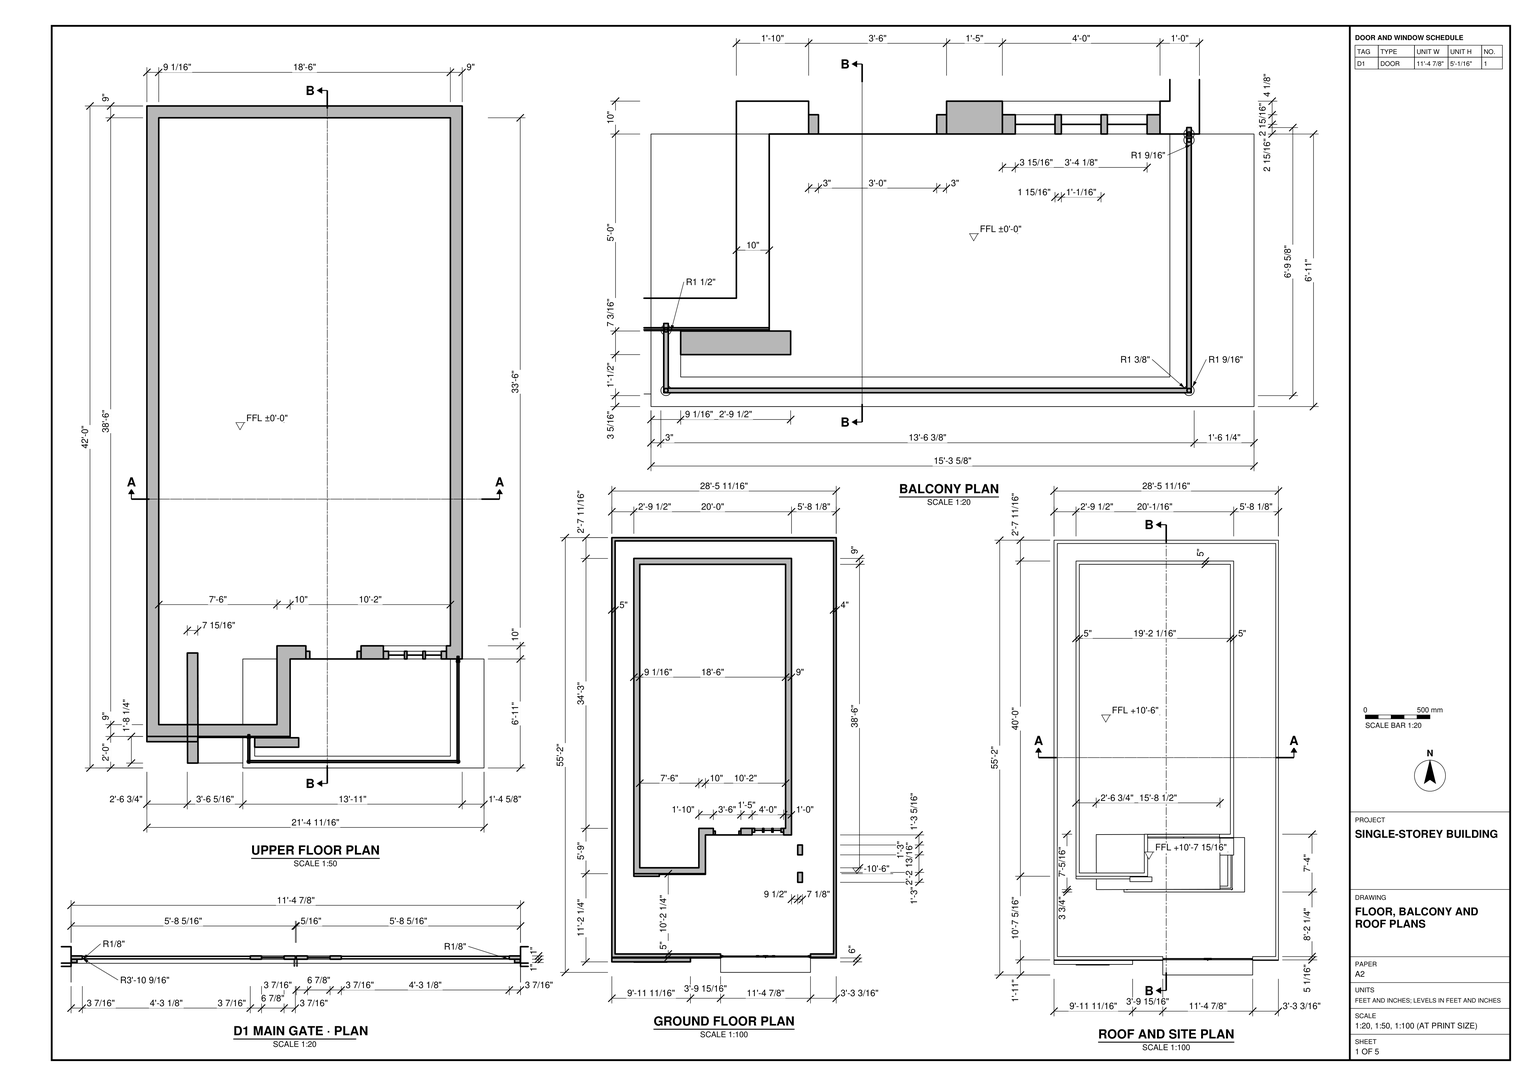
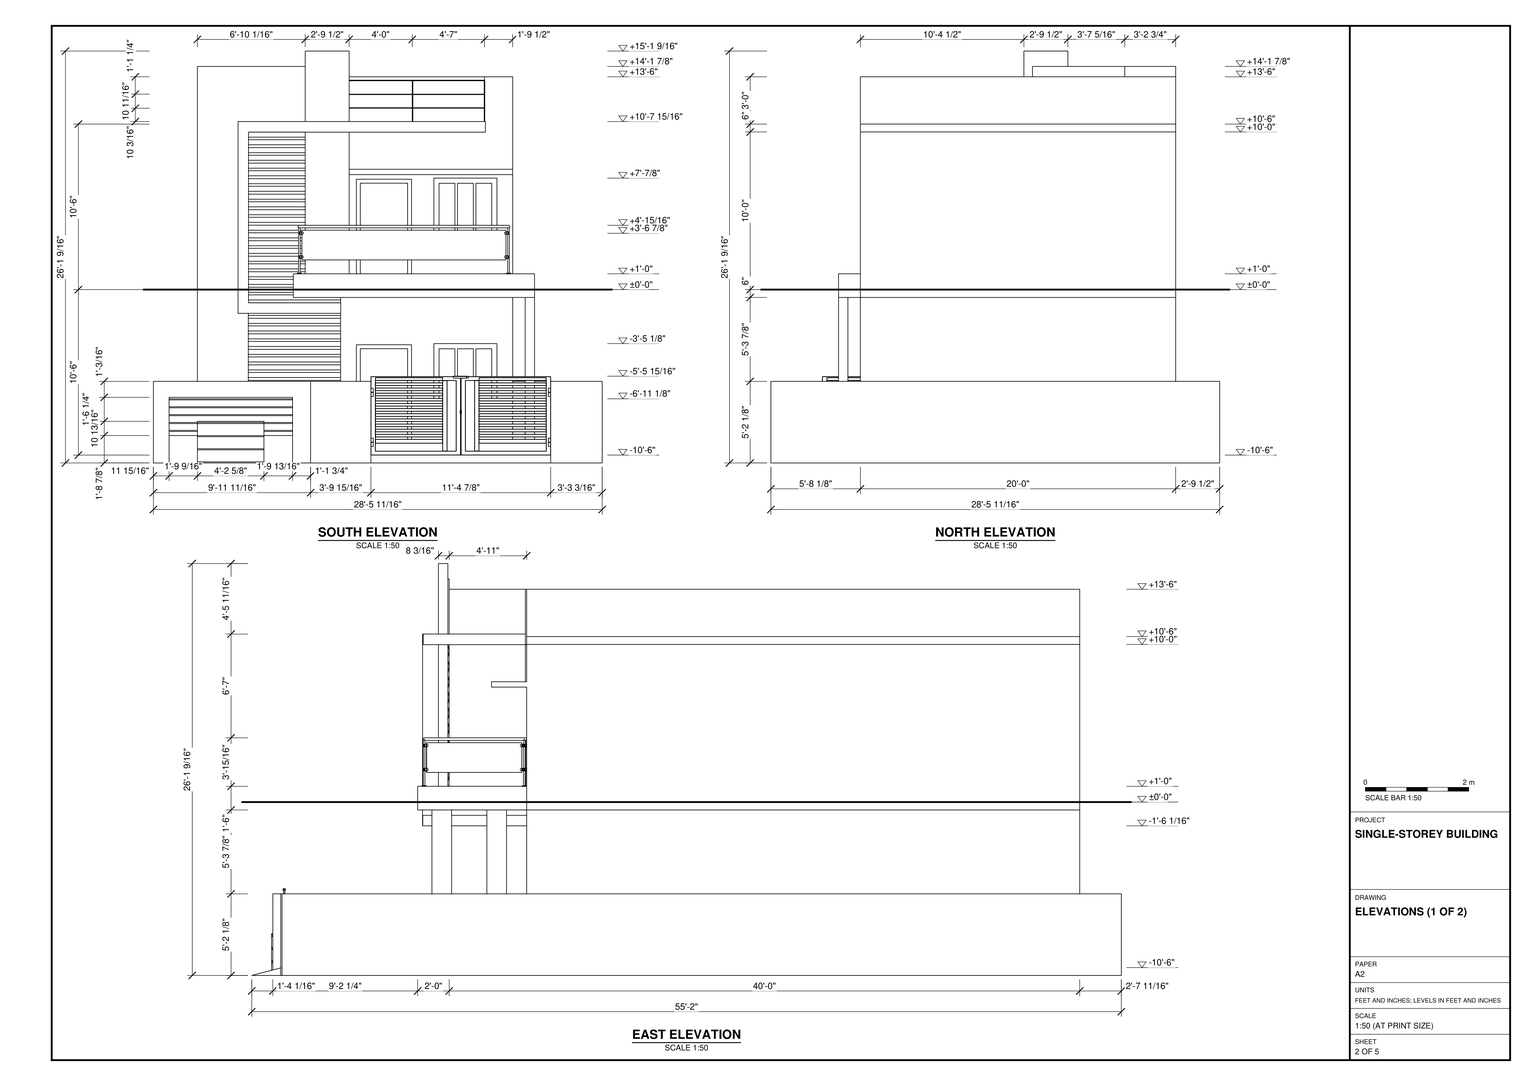
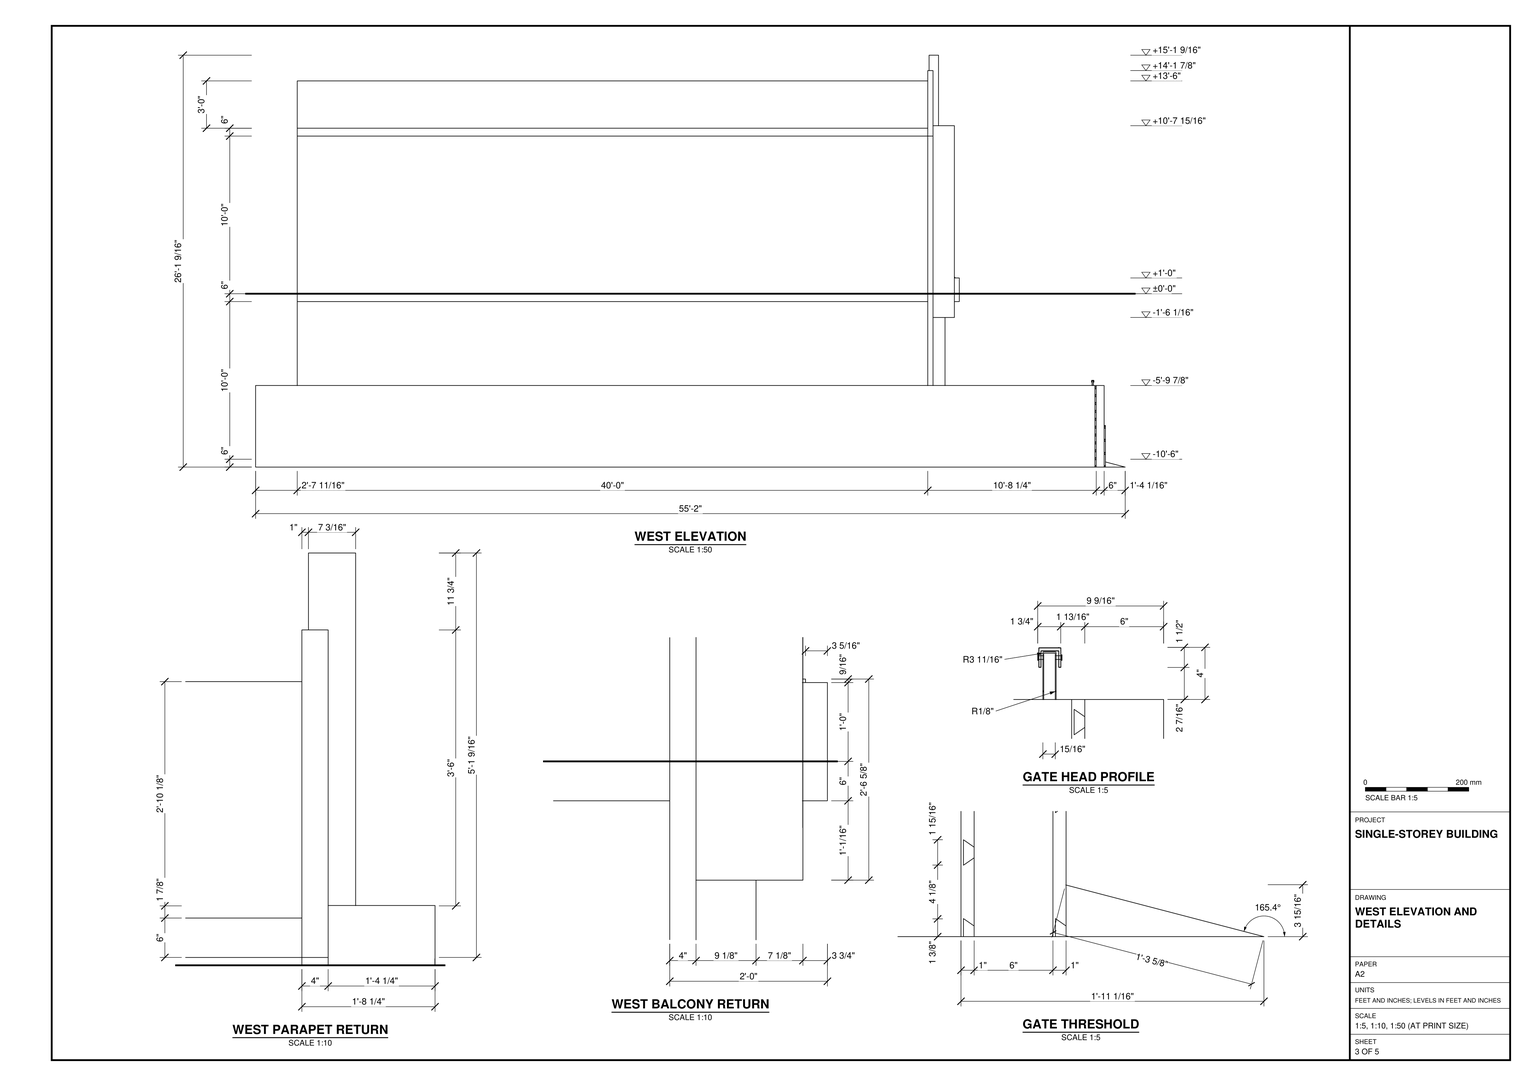
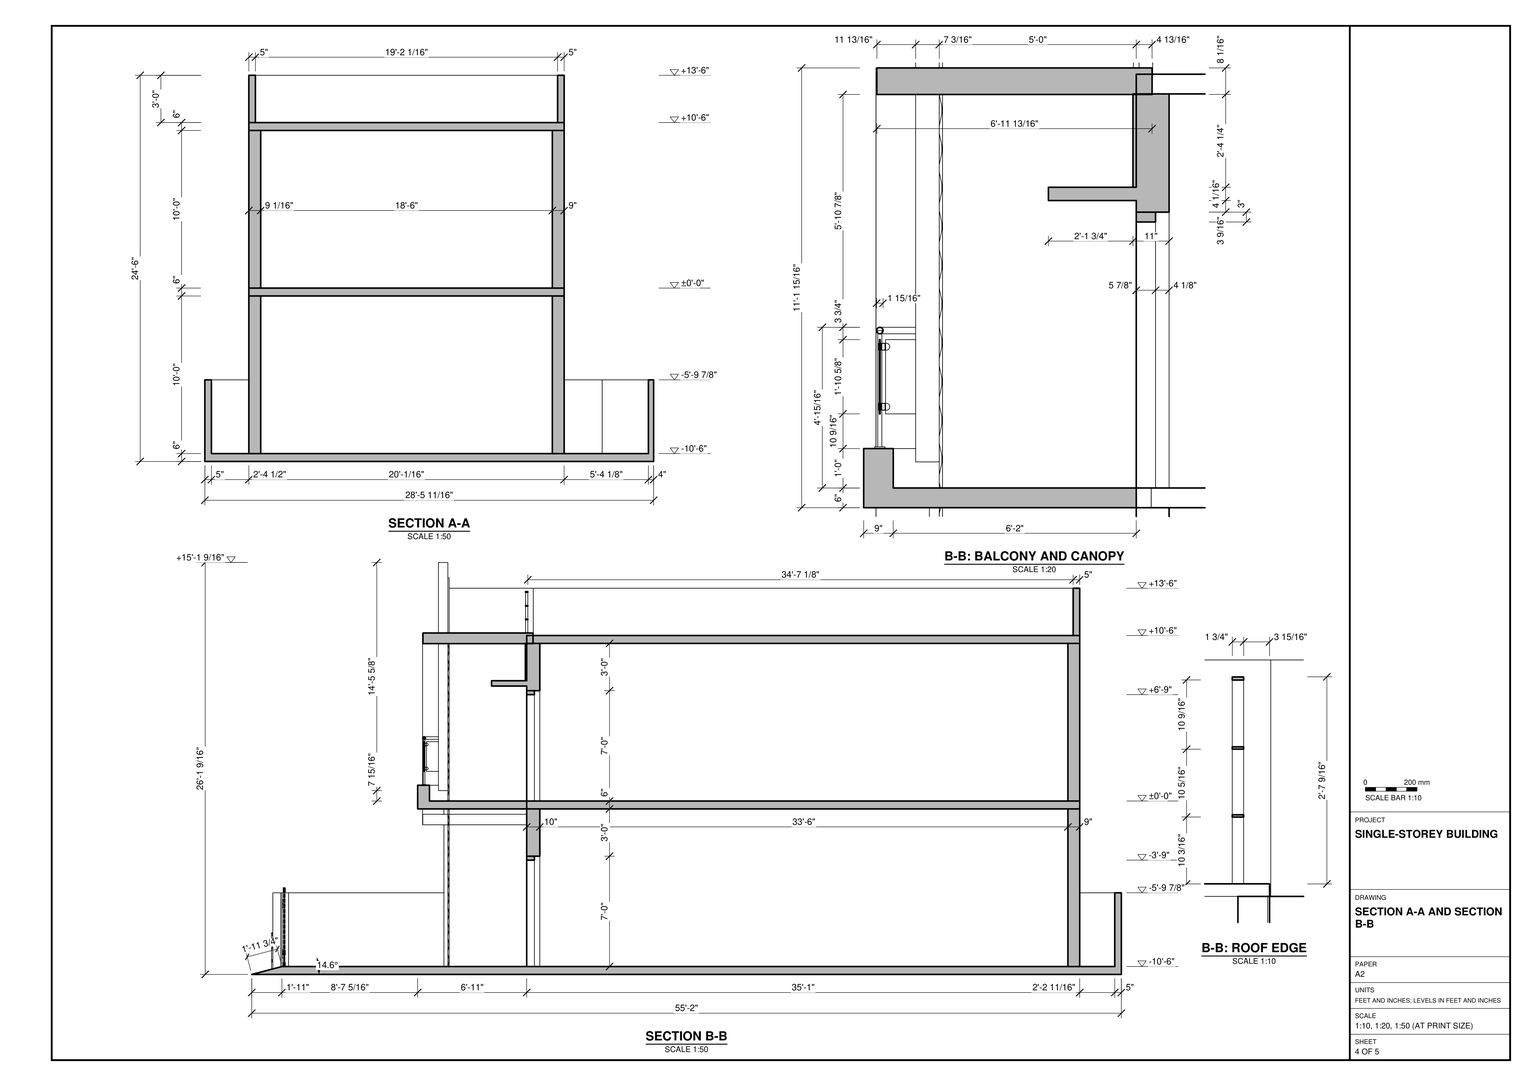
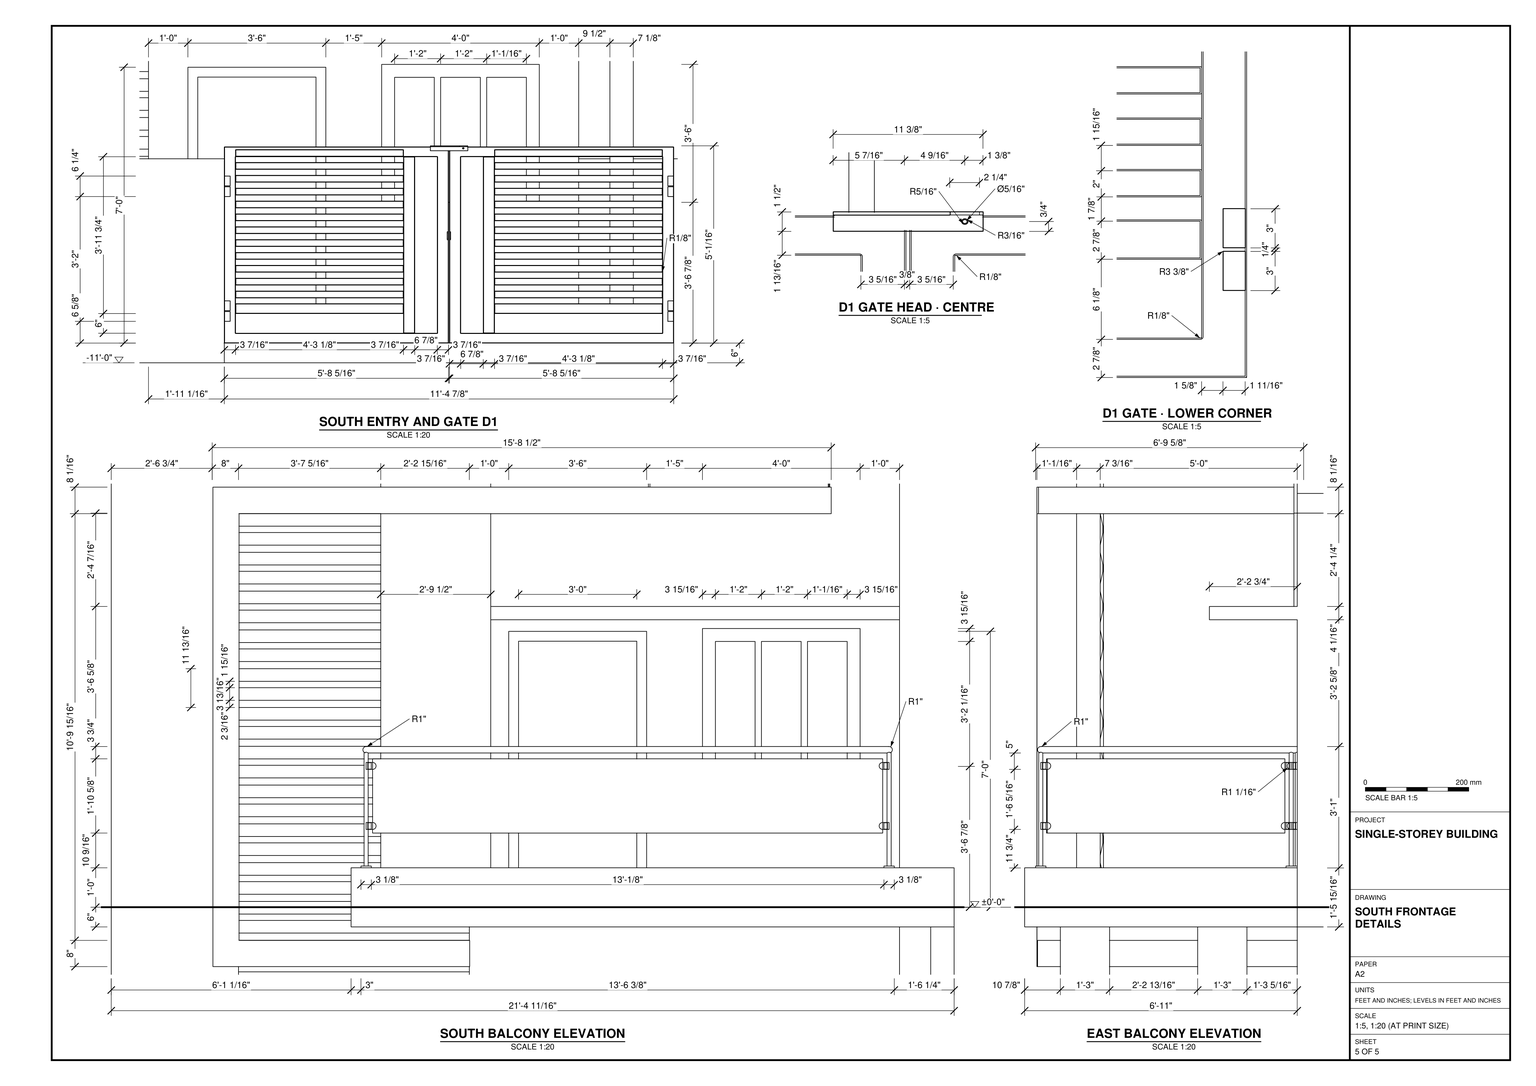
Build the building and its enclosed site in SketchUp from task_files/diagram_01.pdf. Work in feet and inches. The complete model, including the site walls and gate threshold, is 28'-5 11/16" wide, 55'-2" deep and 26'-1 9/16" high. Use the finished floor marked ±0'-0" on the upper floor and balcony plans as the level reference. Set the lower floor, roof slab and parapets relative to that reference as shown in the elevations.

Lay out the building within the site using the side and rear setbacks on the plan. Follow the stepped south wall line and the wall thicknesses drawn for each part of the shell. Model the floor slabs, framed door and window openings, projecting balcony slab, supports and balcony guard with its side returns. Use the south elevation to align the openings on the two floors and to place the horizontally banded facade panel, projecting roof frame and raised parapet feature. At the south site wall, include the patterned wall panel, paired gate leaves, hinges and sloped threshold.

Keep shell elements such as walls, slabs and roof, and each furniture or joinery piece shown, in separate groups or components. Use components for repeated parts. Decor and loose items, where shown, may be any suitable library components. Save one SketchUp model as output_files/building_front_balcony_and_gated_enclosure.skp.

# SketchUp Ruby script. Lengths in inches.
U = 1.inch
M = Sketchup.active_model
def pt(a) = Geom::Point3d.new(a.map { |v| v * U })
def face(e, loops, mat)
  f = e.add_face(loops[0].map { |a| pt(a) })
  loops[1..].each { |l| e.add_face(l.map { |a| pt(a) }).erase! }
  f.material = f.back_material = mat if mat
  f
end
# faces: each face lists its corners as indices into pts; further lists are holes
def faces(e, pts, list, mat = nil) = list.each { |f| face(e, (f[0].is_a?(Array) ? f : [f]).map { |l| l.map { |i| pts[i] } }, mat) }
# xy, xz, yz: faces in a plane at the given z, y or x. An outline is a flat list of corners, or four numbers for a rectangle; further outlines are holes
def ring(l) = l.size == 4 ? [[l[0], l[1]], [l[2], l[1]], [l[2], l[3]], [l[0], l[3]]] : l.each_slice(2).to_a
def flat(e, list, mat, &to3) = list.each { |f| face(e, (f[0].is_a?(Array) ? f : [f]).map { |l| ring(l).map { |u, v| to3.(u, v) } }, mat) }
def xy(e, z, list, mat = nil) = flat(e, list, mat) { |x, y| [x, y, z] }
def xz(e, y, list, mat = nil) = flat(e, list, mat) { |x, z| [x, y, z] }
def yz(e, x, list, mat = nil) = flat(e, list, mat) { |y, z| [x, y, z] }
def lines(e, pts, list) = list.each { |a, b| e.add_line(pt(pts[a]), pt(pts[b])) }
# prism: a flat outline (further loops are holes) pulled along v
def prism(e, loops, v, mat = nil)
  f = face(e, loops, mat); d = Geom::Vector3d.new(v.map { |x| x * U })
  f.pushpull(f.normal.samedirection?(d) ? d.length : -d.length)
end
def box(e, o, s, mat = nil) = prism(e, [[o, [o[0] + s[0], o[1], o[2]], [o[0] + s[0], o[1] + s[1], o[2]], [o[0], o[1] + s[1], o[2]]]], [0, 0, s[2]], mat)
def at(x, y, z, deg = 0) = Geom::Transformation.translation(pt([x, y, z])) * Geom::Transformation.rotation(ORIGIN, Z_AXIS, deg.degrees)
def axes(o, x, y, z) = Geom::Transformation.new([*x, 0, *y, 0, *z, 0, *pt(o).to_a, 1])
def part(name) = M.definitions.add(name)
# library, detail: a bought-in or finely detailed component or shape, given as its bounding box
def library(name, o, s) = part(name).tap { |d| box(d.entities, o, s) }
def detail(e, o, s) = box(e.add_group.entities, o, s)
def put(e, d, t, mat = nil) = e.add_instance(d, t).tap { |i| i.material = mat if mat }
def group(e, t, mat = nil) = e.add_group.tap { |g| g.transformation = t; g.material = mat if mat }.entities
root = M.entities
M.materials.add("[Cladding Siding White]").color = [207, 207, 207]
M.materials.add("[Cladding Stucco White]").color = [200, 200, 200]
M.materials.add("[Color D01]").color = [255, 242, 204]
M.materials.add("[Color D06]").color = [204, 153, 0]
M.materials.add("[Color E01]").color = [255, 255, 204]
M.materials.add("[Color E03]").color = [255, 255, 101]
M.materials.add("[Concrete Form 4x8]").color = [167, 170, 168]
M.materials.add("[Roofing Shingles Variable]").color = [147, 122, 106]
M.materials.add("[Tile Hexagon White]").color = [213, 206, 204]
M.materials.add("[Wood Cherry Original]").color = [152, 86, 42]
M.materials.add("[Wood Veneer 01]").color = [120, 70, 37]
c1 = part("Rectangular column")
box(c1.entities,[-3.375,0,0],[7.125,15,120])
c2 = library("Main Gate",[0,-1.74,0],[119.75,5.32,60.06])
c3 = part("Group5\#2")
xy(c3.entities,0,[[0,0,12.08,38.0625]])
c4 = part("Group3\#2")
xy(c4.entities,0,[[0,0,0,42,48,42,48,0,44.0625,0,44.0625,38.0625,31.98,38.0625,31.98,0,30.04,0,30.04,38.0625,17.96,38.0625,17.96,0,16.02,0,16.02,38.0625,3.9375,38.0625,3.9375,0]])
xy(c4.entities,5.875,[[0,0,3.9375,0,3.9375,38.0625,16.02,38.0625,16.02,0,17.96,0,17.96,38.0625,30.04,38.0625,30.04,0,31.98,0,31.98,38.0625,44.0625,38.0625,44.0625,0,48,0,48,42,0,42]],"[Wood Veneer 01]")
xz(c4.entities,0,[[0,0,3.9375,5.875],[16.02,0,17.96,5.875],[30.04,0,31.98,5.875],[44.0625,0,48,5.875]])
xz(c4.entities,38.0625,[[3.9375,0,16.02,5.875],[17.96,0,30.04,5.875],[31.98,0,44.0625,5.875]])
xz(c4.entities,42,[[0,0,48,5.875]])
yz(c4.entities,0,[[0,0,42,5.875]])
yz(c4.entities,3.9375,[[0,0,38.0625,5.875]])
yz(c4.entities,16.02,[[0,0,38.0625,5.875]])
yz(c4.entities,17.96,[[0,0,38.0625,5.875]])
yz(c4.entities,30.04,[[0,0,38.0625,5.875]])
yz(c4.entities,31.98,[[0,0,38.0625,5.875]])
yz(c4.entities,44.0625,[[0,0,38.0625,5.875]])
yz(c4.entities,48,[[0,0,42,5.875]])
p = [[44.0625,0,0],[31.98,0,0],[16.02,0,0],[3.9375,0,0],[30.04,0,0],[17.96,0,0],
  [0.08,0.08,0],[0.08,0.08,5.875]]
lines(c4.entities,p,[[0,1],[2,3],[4,5],[6,7]])
put(c4.entities,c3,at(3.9375,0,2.9375))
put(c4.entities,c3,at(17.96,0,2.9375))
put(c4.entities,c3,at(31.98,0,2.9375))
c5 = part("Group5\#1")
xy(c5.entities,0,[[-21,-42,-21,42,21,42,21,-42,18,-42,18,39,-18,39,-18,-42]])
xy(c5.entities,5.875,[[-21,-42,-18,-42,-18,39,18,39,18,-42,21,-42,21,42,-21,42]],"[Wood Veneer 01]")
xz(c5.entities,-42,[[-21,0,-18,5.875],[18,0,21,5.875]])
xz(c5.entities,39,[[-18,0,18,5.875]])
xz(c5.entities,42,[[-21,0,21,5.875]])
yz(c5.entities,-21,[[-42,0,42,5.875]])
yz(c5.entities,-18,[[-42,0,39,5.875]])
yz(c5.entities,18,[[-42,0,39,5.875]])
yz(c5.entities,21,[[-42,0,42,5.875]])
c6 = part("Group3\#1")
xy(c6.entities,0,[[0,0,0,42,48,42,48,0,44.0625,0,44.0625,38.0625,31.98,38.0625,31.98,0,30.04,0,30.04,38.0625,17.96,38.0625,17.96,0,16.02,0,16.02,38.0625,3.9375,38.0625,3.9375,0]])
xy(c6.entities,5.875,[[0,0,3.9375,0,3.9375,38.0625,16.02,38.0625,16.02,0,17.96,0,17.96,38.0625,30.04,38.0625,30.04,0,31.98,0,31.98,38.0625,44.0625,38.0625,44.0625,0,48,0,48,42,0,42]],"[Wood Veneer 01]")
xz(c6.entities,0,[[0,0,3.9375,5.875],[16.02,0,17.96,5.875],[30.04,0,31.98,5.875],[44.0625,0,48,5.875]])
xz(c6.entities,38.0625,[[3.9375,0,16.02,5.875],[17.96,0,30.04,5.875],[31.98,0,44.0625,5.875]])
xz(c6.entities,42,[[0,0,48,5.875]])
yz(c6.entities,0,[[0,0,42,5.875]])
yz(c6.entities,3.9375,[[0,0,38.0625,5.875]])
yz(c6.entities,16.02,[[0,0,38.0625,5.875]])
yz(c6.entities,17.96,[[0,0,38.0625,5.875]])
yz(c6.entities,30.04,[[0,0,38.0625,5.875]])
yz(c6.entities,31.98,[[0,0,38.0625,5.875]])
yz(c6.entities,44.0625,[[0,0,38.0625,5.875]])
yz(c6.entities,48,[[0,0,42,5.875]])
p = [[44.0625,0,0],[31.98,0,0],[16.02,0,0],[3.9375,0,0],[30.04,0,0],[17.96,0,0],
  [0.08,0.08,0],[0.08,0.08,5.875]]
lines(c6.entities,p,[[0,1],[2,3],[4,5],[6,7]])
put(c6.entities,c3,at(3.9375,0,2.9375))
put(c6.entities,c3,at(17.96,0,2.9375))
put(c6.entities,c3,at(31.98,0,2.9375))
c7 = part("Group5\#3")
xy(c7.entities,0,[[-21,-42,-21,42,21,42,21,-42,18,-42,18,39,-18,39,-18,-42]])
xy(c7.entities,5.875,[[-21,-42,-18,-42,-18,39,18,39,18,-42,21,-42,21,42,-21,42]],"[Wood Veneer 01]")
xz(c7.entities,-42,[[-21,0,-18,5.875],[18,0,21,5.875]])
xz(c7.entities,39,[[-18,0,18,5.875]])
xz(c7.entities,42,[[-21,0,21,5.875]])
yz(c7.entities,-21,[[-42,0,42,5.875]])
yz(c7.entities,-18,[[-42,0,39,5.875]])
yz(c7.entities,18,[[-42,0,39,5.875]])
yz(c7.entities,21,[[-42,0,42,5.875]])
c8 = library("Group\#7",[0,0,0],[70.28,1,246])
c9 = library("Group\#12",[0,0,0],[162.4,81.63,36.98])
c10 = part("Group18\#1")
box(c10.entities,[218.29,58.13,253.91],[0.47,1.74,31.03])
c11 = part("Group19\#1")
box(c11.entities,[108.76,58.13,253.91],[0.48,1.74,31.03])
c12 = part("Group20\#1")
box(c12.entities,[163.53,58.13,253.91],[0.47,1.74,31.03])
c13 = part("Group21\#1")
box(c13.entities,[108.76,58.13,284.94],[110,1.74,0.47])
c14 = part("Group22\#1")
box(c14.entities,[109,58.13,264.08],[109.53,1.74,0.35])
box(c14.entities,[109,58.13,274.42],[109.53,1.74,0.35])
xz(root,209.3125,[[157.53,0,193.53,81],[157.53,126,193.53,207]],"[Wood Cherry Original]")
p = [[142.53,214.3125,252],[252.59,214.3125,252],[142.53,202.15,252],[165.47,202.15,252],[175.47,202.15,252]]
lines(root,p,[[0,1],[2,3],[3,4]])
put(root,c1,at(286.41,179,0),"[Color E01]")
put(root,c1,at(286.41,137.18,0),"[Color E01]")
put(root,c2,axes([165.61,23.24,0],[1.14289,0,0],[0,0.67255,0],[0,0,1]))
put(root,c4,axes([213.53,219.3125,42.86],[1,0,0],[0,0,1],[0,-1,0]))
put(root,c5,axes([175.53,215.1875,42],[1,0,0],[0,0,1],[0,-1,0]))
g1 = group(root,at(33.5,150.32,0),"[Color E01]")
xy(g1,0,[[0,0,0,480,240.03,480,240.03,59,163.03,59,163.03,69,231.03,69,231.03,471,9.03,471,9.03,9,99.03,9,99.03,69,121.03,69,121.03,59,109.03,59,109.03,0],[9.03,9,9.03,471,231.03,471,231.03,69,163.03,69,163.03,59,121.03,59,121.03,69,99.03,69,99.03,9]])
xy(g1,42.86,[[180.03,59,228.03,69]])
xy(g1,84,[[121.03,59,163.03,69]])
xy(g1,84.86,[[180.03,59,228.03,69]])
xy(g1,120,[[[0,0,109.03,0,109.03,59,240.03,59,240.03,480,0,480],[9.03,9,9.03,471,231.03,471,231.03,69,99.03,69,99.03,9]]])
xz(g1,0,[[0,0,109.03,120]])
xz(g1,9,[[9.03,0,99.03,120]])
xz(g1,59,[[[109.03,0,121.03,0,121.03,84,163.03,84,163.03,0,240.03,0,240.03,120,109.03,120],[180.03,42.86,228.03,84.86]]])
xz(g1,69,[[[99.03,0,99.03,120,231.03,120,231.03,0,163.03,0,163.03,84,121.03,84,121.03,0],[180.03,42.86,228.03,84.86]]])
xz(g1,471,[[9.03,0,231.03,120]])
xz(g1,480,[[0,0,240.03,120]])
yz(g1,0,[[0,0,480,120]])
yz(g1,9.03,[[9,0,471,120]])
yz(g1,99.03,[[9,0,69,120]])
yz(g1,109.03,[[0,0,59,120]])
yz(g1,121.03,[[59,0,69,84]])
yz(g1,163.03,[[59,0,69,84]])
yz(g1,180.03,[[59,42.86,69,84.86]])
yz(g1,228.03,[[59,42.86,69,84.86]])
yz(g1,231.03,[[69,0,471,120]])
yz(g1,240.03,[[59,0,480,120]])
p = [[124.03,59,0],[124.03,59,81],[160.03,59,81],[160.03,59,0]]
lines(g1,p,[[0,1],[1,2],[2,3]])
put(root,c6,axes([213.53,215.1875,168.86],[1,0,0],[0,0,1],[0,-1,0]))
put(root,c7,axes([175.53,215.1875,168],[1,0,0],[0,0,1],[0,-1,0]))
g2 = group(root,at(33.5,150.32,120),"[Color E01]")
prism(g2,[[[0,0,0],[0,480,0],[240.03,480,0],[240.03,59,0],[109.03,59,0],[109.03,0,0]]],[0,0,6])
g3 = group(root,at(106.53,126.32,120),"[Color E01]")
xy(g3,0,[[[0,0,183.625,83],[138.28,56.63,139.32,56.71,140.31,57.0625,141.17,57.66,141.84,58.45,142.29,59.39,142.48,60.42,142.39,61.46,142.04,62.45,141.45,63.31,140.65,63.98,139.71,64.43,138.68,64.62,137.64,64.53,136.66,64.18,135.8,63.59,135.125,62.79,134.68,61.85,134.49,60.82,134.57,59.78,134.92,58.8,135.52,57.94,136.3125,57.26,137.25,56.82],[76.33,57.16,77.37,57.27,78.34,57.64,79.18,58.26,79.84,59.07,80.26,60.03,80.43,61.06,80.32,62.1,79.94,63.07,79.33,63.91,78.51,64.57,77.56,64.99,76.53,65.16,75.49,65.05,74.52,64.67,73.67,64.06,73.01,63.24,72.59,62.29,72.43,61.26,72.54,60.22,72.91,59.24,73.53,58.4,74.34,57.74,75.3,57.32],[134.01,24.36,135.05,24.4,136.05,24.71,136.93,25.27,137.64,26.04,138.13,26.96,138.36,27.98,138.32,29.03,138.01,30.02,137.45,30.91,136.68,31.61,135.76,32.1,134.74,32.33,133.7,32.29,132.7,31.98,131.82,31.42,131.11,30.65,130.62,29.73,130.39,28.71,130.43,27.67,130.74,26.67,131.3,25.79,132.07,25.08,132.99,24.59],[75.3125,24.98,76.33,25.22,77.24,25.73,78,26.45,78.54,27.34,78.83,28.34,78.85,29.39,78.6,30.4,78.1,31.32,77.38,32.07,76.49,32.61,75.49,32.91,74.44,32.93,73.43,32.68,72.51,32.18,71.76,31.46,71.22,30.5625,70.92,29.5625,70.9,28.52,71.15,27.5,71.65,26.59,72.375,25.83,73.27,25.29,74.27,25]]])
xy(g3,2.3125,[[134.01,24.36,132.99,24.59,132.07,25.08,131.3,25.79,130.74,26.67,130.43,27.67,130.39,28.71,130.62,29.73,131.11,30.65,131.82,31.42,132.7,31.98,133.7,32.29,134.74,32.33,135.76,32.1,136.68,31.61,137.45,30.91,138.01,30.02,138.32,29.03,138.36,27.98,138.13,26.96,137.64,26.04,136.93,25.27,136.05,24.71,135.05,24.4],[75.3125,24.98,74.27,25,73.27,25.29,72.375,25.83,71.65,26.59,71.15,27.5,70.9,28.52,70.92,29.5625,71.22,30.5625,71.76,31.46,72.51,32.18,73.43,32.68,74.44,32.93,75.49,32.91,76.49,32.61,77.38,32.07,78.1,31.32,78.6,30.4,78.85,29.39,78.83,28.34,78.54,27.34,78,26.45,77.24,25.73,76.33,25.22],[138.28,56.63,137.25,56.82,136.3125,57.26,135.52,57.94,134.92,58.8,134.57,59.78,134.49,60.82,134.68,61.85,135.125,62.79,135.8,63.59,136.66,64.18,137.64,64.53,138.68,64.62,139.71,64.43,140.65,63.98,141.45,63.31,142.04,62.45,142.39,61.46,142.48,60.42,142.29,59.39,141.84,58.45,141.17,57.66,140.31,57.0625,139.32,56.71],[76.33,57.16,75.3,57.32,74.34,57.74,73.53,58.4,72.91,59.24,72.54,60.22,72.43,61.26,72.59,62.29,73.01,63.24,73.67,64.06,74.52,64.67,75.49,65.05,76.53,65.16,77.56,64.99,78.51,64.57,79.33,63.91,79.94,63.07,80.32,62.1,80.43,61.06,80.26,60.03,79.84,59.07,79.18,58.26,78.34,57.64,77.37,57.27]],"[Color E03]")
xy(g3,6,[[9.04,9,158,9,158,83,0,83,0,24,9.04,24]])
xy(g3,18,[[0,0,183.625,0,183.625,83,158,83,158,9,9.04,9,9.04,24,0,24]])
xz(g3,0,[[0,0,183.625,18]])
xz(g3,9,[[9.04,6,158,18]])
xz(g3,24,[[0,6,9.04,18]])
xz(g3,83,[[0,0,0,6,158,6,158,18,183.625,18,183.625,0]])
yz(g3,0,[[0,0,0,18,24,18,24,6,83,6,83,0]])
yz(g3,9.04,[[9,6,24,18]])
yz(g3,158,[[9,6,83,18]])
yz(g3,183.625,[[0,0,83,18]])
p = [[134.01,24.36,0],[132.99,24.59,0],[132.99,24.59,2.3125],[134.01,24.36,2.3125],[135.05,24.4,0],[135.05,24.4,2.3125],
  [136.05,24.71,0],[136.05,24.71,2.3125],[132.07,25.08,0],[132.07,25.08,2.3125],[136.93,25.27,0],[136.93,25.27,2.3125],
  [74.27,25,0],[73.27,25.29,0],[73.27,25.29,2.3125],[74.27,25,2.3125],[75.3125,24.98,0],[75.3125,24.98,2.3125],
  [76.33,25.22,0],[76.33,25.22,2.3125],[131.3,25.79,0],[131.3,25.79,2.3125],[77.24,25.73,0],[77.24,25.73,2.3125],
  [72.375,25.83,0],[72.375,25.83,2.3125],[137.64,26.04,0],[137.64,26.04,2.3125],[78,26.45,0],[78,26.45,2.3125],
  [71.65,26.59,0],[71.65,26.59,2.3125],[130.74,26.67,0],[130.74,26.67,2.3125],[138.13,26.96,0],[138.13,26.96,2.3125],
  [78.54,27.34,0],[78.54,27.34,2.3125],[71.15,27.5,0],[71.15,27.5,2.3125],[130.43,27.67,0],[130.43,27.67,2.3125],
  [138.36,27.98,0],[138.36,27.98,2.3125],[78.83,28.34,0],[78.83,28.34,2.3125],[70.9,28.52,0],[70.9,28.52,2.3125],
  [130.39,28.71,0],[130.39,28.71,2.3125],[138.32,29.03,0],[138.32,29.03,2.3125],[78.85,29.39,0],[78.85,29.39,2.3125],
  [70.92,29.5625,0],[70.92,29.5625,2.3125],[130.62,29.73,0],[130.62,29.73,2.3125],[138.01,30.02,0],[138.01,30.02,2.3125],
  [78.6,30.4,0],[78.6,30.4,2.3125],[71.22,30.5625,0],[71.22,30.5625,2.3125],[131.11,30.65,0],[131.11,30.65,2.3125],
  [137.45,30.91,0],[137.45,30.91,2.3125],[78.1,31.32,0],[78.1,31.32,2.3125],[71.76,31.46,0],[71.76,31.46,2.3125],
  [131.82,31.42,0],[131.82,31.42,2.3125],[136.68,31.61,0],[136.68,31.61,2.3125],[77.38,32.07,0],[77.38,32.07,2.3125],
  [132.7,31.98,0],[132.7,31.98,2.3125],[72.51,32.18,0],[72.51,32.18,2.3125],[135.76,32.1,0],[135.76,32.1,2.3125],
  [133.7,32.29,0],[133.7,32.29,2.3125],[76.49,32.61,0],[76.49,32.61,2.3125],[134.74,32.33,0],[134.74,32.33,2.3125],
  [73.43,32.68,0],[73.43,32.68,2.3125],[75.49,32.91,0],[75.49,32.91,2.3125],[74.44,32.93,0],[74.44,32.93,2.3125],
  [138.28,56.63,0],[137.25,56.82,0],[137.25,56.82,2.3125],[138.28,56.63,2.3125],[139.32,56.71,0],[139.32,56.71,2.3125],
  [140.31,57.0625,0],[140.31,57.0625,2.3125],[136.3125,57.26,0],[136.3125,57.26,2.3125],[141.17,57.66,0],[141.17,57.66,2.3125],
  [76.33,57.16,0],[75.3,57.32,0],[75.3,57.32,2.3125],[76.33,57.16,2.3125],[77.37,57.27,0],[77.37,57.27,2.3125],
  [74.34,57.74,0],[74.34,57.74,2.3125],[78.34,57.64,0],[78.34,57.64,2.3125],[135.52,57.94,0],[135.52,57.94,2.3125],
  [79.18,58.26,0],[79.18,58.26,2.3125],[73.53,58.4,0],[73.53,58.4,2.3125],[141.84,58.45,0],[141.84,58.45,2.3125],
  [134.92,58.8,0],[134.92,58.8,2.3125],[79.84,59.07,0],[79.84,59.07,2.3125],[72.91,59.24,0],[72.91,59.24,2.3125],
  [142.29,59.39,0],[142.29,59.39,2.3125],[134.57,59.78,0],[134.57,59.78,2.3125],[80.26,60.03,0],[80.26,60.03,2.3125],
  [72.54,60.22,0],[72.54,60.22,2.3125],[142.48,60.42,0],[142.48,60.42,2.3125],[134.49,60.82,0],[134.49,60.82,2.3125],
  [80.43,61.06,0],[80.43,61.06,2.3125],[72.43,61.26,0],[72.43,61.26,2.3125],[142.39,61.46,0],[142.39,61.46,2.3125],
  [134.68,61.85,0],[134.68,61.85,2.3125],[80.32,62.1,0],[80.32,62.1,2.3125],[72.59,62.29,0],[72.59,62.29,2.3125],
  [142.04,62.45,0],[142.04,62.45,2.3125],[135.125,62.79,0],[135.125,62.79,2.3125],[79.94,63.07,0],[79.94,63.07,2.3125],
  [73.01,63.24,0],[73.01,63.24,2.3125],[141.45,63.31,0],[141.45,63.31,2.3125],[135.8,63.59,0],[135.8,63.59,2.3125],
  [79.33,63.91,0],[79.33,63.91,2.3125],[73.67,64.06,0],[73.67,64.06,2.3125],[140.65,63.98,0],[140.65,63.98,2.3125],
  [136.66,64.18,0],[136.66,64.18,2.3125],[78.51,64.57,0],[78.51,64.57,2.3125],[139.71,64.43,0],[139.71,64.43,2.3125],
  [74.52,64.67,0],[74.52,64.67,2.3125],[137.64,64.53,0],[137.64,64.53,2.3125],[138.68,64.62,0],[138.68,64.62,2.3125],
  [77.56,64.99,0],[77.56,64.99,2.3125],[75.49,65.05,0],[75.49,65.05,2.3125],[76.53,65.16,0],[76.53,65.16,2.3125]]
faces(g3,p,[[0,1,2,3],[4,0,3,5],[6,4,5,7],[1,8,9,2],[10,6,7,11],[12,13,14,15],[16,12,15,17],[18,16,17,19],
  [8,20,21,9],[22,18,19,23],[13,24,25,14],[26,10,11,27],[28,22,23,29],[24,30,31,25],[20,32,33,21],[34,26,27,35],
  [36,28,29,37],[30,38,39,31],[32,40,41,33],[42,34,35,43],[44,36,37,45],[38,46,47,39],[40,48,49,41],[50,42,43,51],
  [52,44,45,53],[46,54,55,47],[48,56,57,49],[58,50,51,59],[60,52,53,61],[54,62,63,55],[56,64,65,57],[66,58,59,67],
  [68,60,61,69],[62,70,71,63],[64,72,73,65],[74,66,67,75],[76,68,69,77],[72,78,79,73],[70,80,81,71],[82,74,75,83],
  [78,84,85,79],[86,76,77,87],[88,82,83,89],[80,90,91,81],[84,88,89,85],[92,86,87,93],[90,94,95,91],[94,92,93,95],
  [96,97,98,99],[100,96,99,101],[102,100,101,103],[97,104,105,98],[106,102,103,107],[108,109,110,111],[112,108,111,113],[109,114,115,110],
  [116,112,113,117],[104,118,119,105],[120,116,117,121],[114,122,123,115],[124,106,107,125],[118,126,127,119],[128,120,121,129],[122,130,131,123],
  [132,124,125,133],[126,134,135,127],[136,128,129,137],[130,138,139,131],[140,132,133,141],[134,142,143,135],[144,136,137,145],[138,146,147,139],
  [148,140,141,149],[142,150,151,143],[152,144,145,153],[146,154,155,147],[156,148,149,157],[150,158,159,151],[160,152,153,161],[154,162,163,155],
  [164,156,157,165],[158,166,167,159],[168,160,161,169],[162,170,171,163],[172,164,165,173],[166,174,175,167],[176,168,169,177],[178,172,173,179],
  [170,180,181,171],[174,182,183,175],[184,178,179,185],[182,184,185,183],[186,176,177,187],[180,188,189,181],[188,190,191,189],[190,186,187,191]],"[Color E03]")
put(root,c8,at(72.25,149.32,0),"[Wood Veneer 01]")
g4 = group(root,at(64.26,130.04,107.91),"[Color D01]")
xy(g4,0,[[0.2,0,-0.02,83.81,78.16,84.01,78.39,0.21]])
xy(g4,7.98,[[8.16,0.02,78.39,0.21,78.16,84.01,7.94,83.83]])
xy(g4,137.92,[[[8.16,0.02,7.94,83.83,188.24,84.3,188.46,0.5],[111.52,32.04,112.56,32.18,113.52,32.58,114.35,33.21,114.98,34.04,115.38,35.01,115.52,36.04,115.38,37.08,114.98,38.04,114.35,38.87,113.52,39.51,112.56,39.91,111.52,40.04,110.49,39.91,109.52,39.51,108.69,38.87,108.06,38.04,107.66,37.08,107.52,36.04,107.66,35.01,108.06,34.04,108.69,33.21,109.52,32.58,110.49,32.18],[159.82,32.44,160.83,32.71,161.73,33.23,162.47,33.96,163,34.86,163.28,35.87,163.28,36.91,163.01,37.92,162.5,38.83,161.76,39.57,160.86,40.1,159.85,40.375,158.81,40.38,157.8,40.11,156.89,39.59,156.15,38.86,155.625,37.96,155.35,36.95,155.34,35.91,155.61,34.9,156.13,33.99,156.86,33.25,157.77,32.72,158.77,32.45]]])
xy(g4,139.67,[[111.52,32.04,110.49,32.18,109.52,32.58,108.69,33.21,108.06,34.04,107.66,35.01,107.52,36.04,107.66,37.08,108.06,38.04,108.69,38.87,109.52,39.51,110.49,39.91,111.52,40.04,112.56,39.91,113.52,39.51,114.35,38.87,114.98,38.04,115.38,37.08,115.52,36.04,115.38,35.01,114.98,34.04,114.35,33.21,113.52,32.58,112.56,32.18],[159.82,32.44,158.77,32.45,157.77,32.72,156.86,33.25,156.13,33.99,155.61,34.9,155.34,35.91,155.35,36.95,155.625,37.96,156.15,38.86,156.89,39.59,157.8,40.11,158.81,40.38,159.85,40.375,160.86,40.1,161.76,39.57,162.5,38.83,163.01,37.92,163.28,36.91,163.28,35.87,163,34.86,162.47,33.96,161.73,33.23,160.83,32.71]],"[Color E03]")
xy(g4,146,[[0.2,0,188.46,0.5,188.24,84.3,-0.02,83.81]])
yz(g4,163.28,[[35.87,137.92,36.91,139.67]],"[Color E03]")
p = [[-0.02,83.81,146],[-0.02,83.81,0],[0.2,0,0],[0.2,0,146],[78.39,0.21,7.98],[8.16,0.02,7.98],
  [8.16,0.02,137.92],[188.46,0.5,137.92],[188.46,0.5,146],[78.39,0.21,0],[78.16,84.01,0],[78.16,84.01,7.98],
  [7.94,83.83,7.98],[188.24,84.3,146],[188.24,84.3,137.92],[7.94,83.83,137.92],[111.52,32.04,137.92],[110.49,32.18,137.92],
  [110.49,32.18,139.67],[111.52,32.04,139.67],[112.56,32.18,137.92],[112.56,32.18,139.67],[109.52,32.58,137.92],[109.52,32.58,139.67],
  [113.52,32.58,137.92],[113.52,32.58,139.67],[158.77,32.45,137.92],[157.77,32.72,137.92],[157.77,32.72,139.67],[158.77,32.45,139.67],
  [159.82,32.44,137.92],[159.82,32.44,139.67],[160.83,32.71,137.92],[160.83,32.71,139.67],[108.69,33.21,137.92],[108.69,33.21,139.67],
  [114.35,33.21,137.92],[114.35,33.21,139.67],[156.86,33.25,137.92],[156.86,33.25,139.67],[161.73,33.23,137.92],[161.73,33.23,139.67],
  [108.06,34.04,137.92],[108.06,34.04,139.67],[114.98,34.04,137.92],[114.98,34.04,139.67],[156.13,33.99,137.92],[156.13,33.99,139.67],
  [162.47,33.96,137.92],[162.47,33.96,139.67],[107.66,35.01,137.92],[107.66,35.01,139.67],[115.38,35.01,137.92],[115.38,35.01,139.67],
  [155.61,34.9,137.92],[155.61,34.9,139.67],[163,34.86,137.92],[163,34.86,139.67],[155.34,35.91,137.92],[155.34,35.91,139.67],
  [163.28,35.87,137.92],[163.28,35.87,139.67],[107.52,36.04,137.92],[107.52,36.04,139.67],[115.52,36.04,137.92],[115.52,36.04,139.67],
  [155.35,36.95,137.92],[155.35,36.95,139.67],[107.66,37.08,137.92],[107.66,37.08,139.67],[115.38,37.08,137.92],[115.38,37.08,139.67],
  [163.01,37.92,137.92],[163.28,36.91,137.92],[163.28,36.91,139.67],[163.01,37.92,139.67],[155.625,37.96,137.92],[155.625,37.96,139.67],
  [108.06,38.04,137.92],[108.06,38.04,139.67],[114.98,38.04,137.92],[114.98,38.04,139.67],[162.5,38.83,137.92],[162.5,38.83,139.67],
  [108.69,38.87,137.92],[108.69,38.87,139.67],[114.35,38.87,137.92],[114.35,38.87,139.67],[156.15,38.86,137.92],[156.15,38.86,139.67],
  [161.76,39.57,137.92],[161.76,39.57,139.67],[109.52,39.51,137.92],[109.52,39.51,139.67],[113.52,39.51,137.92],[113.52,39.51,139.67],
  [156.89,39.59,137.92],[156.89,39.59,139.67],[110.49,39.91,137.92],[110.49,39.91,139.67],[112.56,39.91,137.92],[112.56,39.91,139.67],
  [157.8,40.11,137.92],[157.8,40.11,139.67],[160.86,40.1,137.92],[160.86,40.1,139.67],[111.52,40.04,137.92],[111.52,40.04,139.67],
  [158.81,40.38,137.92],[158.81,40.38,139.67],[159.85,40.375,137.92],[159.85,40.375,139.67]]
faces(g4,p,[[0,1,2,3],[4,5,6,7,8,3,2,9],[10,11,4,9],[12,11,10,1,0,13,14,15],[12,15,6,5],[14,13,8,7]])
faces(g4,p,[[16,17,18,19],[20,16,19,21],[17,22,23,18],[24,20,21,25],[26,27,28,29],[30,26,29,31],[32,30,31,33],[22,34,35,23],
  [36,24,25,37],[27,38,39,28],[40,32,33,41],[34,42,43,35],[44,36,37,45],[38,46,47,39],[48,40,41,49],[42,50,51,43],
  [52,44,45,53],[46,54,55,47],[56,48,49,57],[54,58,59,55],[60,56,57,61],[50,62,63,51],[64,52,53,65],[58,66,67,59],
  [62,68,69,63],[70,64,65,71],[72,73,74,75],[66,76,77,67],[68,78,79,69],[80,70,71,81],[82,72,75,83],[78,84,85,79],
  [86,80,81,87],[76,88,89,77],[90,82,83,91],[84,92,93,85],[94,86,87,95],[88,96,97,89],[92,98,99,93],[100,94,95,101],
  [96,102,103,97],[104,90,91,105],[98,106,107,99],[106,100,101,107],[102,108,109,103],[110,104,105,111],[108,110,111,109]],"[Color E03]")
g5 = group(root,at(115.57,145.44,140),"[Roofing Shingles Variable]")
box(g5,[0,-3.3125,-6.0625],[33.49,7.1875,173.65])
g6 = group(root,at(33.5,146.32,0))
xy(g6,0,[[0,0,38.75,4]])
xy(g6,246,[[38.75,0,109.03,4]])
xy(g6,295.875,[[0,0,109.03,4]])
xz(g6,0,[[0,0,38.75,0,38.75,246,109.03,246,109.03,295.875,0,295.875]],"[Cladding Siding White]")
xz(g6,4,[[38.75,246,109.03,295.875]])
yz(g6,0,[[0,0,4,246],[0,246,4,295.875]])
yz(g6,38.75,[[0,0,4,246]])
yz(g6,109.03,[[0,246,4,295.875]])
g7 = group(root,at(33.5,150.32,126),"[Color E01]")
xy(g7,0,[[0,0,0,480,240.03,480,240.03,59,163.03,59,163.03,69,231.03,69,231.03,471,9.03,471,9.03,9,99.03,9,99.03,69,121.03,69,121.03,59,109.03,59,109.03,0],[9.03,9,9.03,471,231.03,471,231.03,69,163.03,69,163.03,59,121.03,59,121.03,69,99.03,69,99.03,9]])
xy(g7,42.86,[[180.03,59,228.03,69]])
xy(g7,84,[[121.03,59,163.03,69]])
xy(g7,84.86,[[180.03,59,228.03,69]])
xy(g7,87.53,[[109.03,32.25,240.03,59]])
xy(g7,91.58,[[109.03,32.25,240.03,59]])
xy(g7,120,[[[0,0,109.03,0,109.03,59,240.03,59,240.03,480,0,480],[9.03,9,9.03,471,231.03,471,231.03,69,99.03,69,99.03,9]]])
xz(g7,0,[[0,0,109.03,120]])
xz(g7,9,[[9.03,0,99.03,120]])
xz(g7,32.25,[[109.03,87.53,240.03,91.58]])
xz(g7,59,[[[109.03,0,121.03,0,121.03,84,163.03,84,163.03,0,240.03,0,240.03,87.53,109.03,87.53],[180.03,42.86,228.03,84.86]],[109.03,91.58,240.03,120]])
xz(g7,69,[[[99.03,0,99.03,120,231.03,120,231.03,0,163.03,0,163.03,84,121.03,84,121.03,0],[180.03,42.86,228.03,84.86]]])
xz(g7,471,[[9.03,0,231.03,120]])
xz(g7,480,[[0,0,240.03,120]])
yz(g7,0,[[0,0,480,120]])
yz(g7,9.03,[[9,0,471,120]])
yz(g7,99.03,[[9,0,69,120]])
yz(g7,109.03,[[0,0,59,0,59,87.53,32.25,87.53,32.25,91.58,59,91.58,59,120,0,120]])
yz(g7,121.03,[[59,0,69,84]])
yz(g7,163.03,[[59,0,69,84]])
yz(g7,180.03,[[59,42.86,69,84.86]])
yz(g7,228.03,[[59,42.86,69,84.86]])
yz(g7,231.03,[[69,0,471,120]])
yz(g7,240.03,[[59,0,480,0,480,120,59,120,59,91.58,32.25,91.58,32.25,87.53,59,87.53]])
p = [[124.03,59,0],[124.03,59,81],[160.03,59,81],[160.03,59,0]]
lines(g7,p,[[0,1],[1,2],[2,3]])
g8 = group(root,at(33.5,150.32,252),"[Color E01]")
xy(g8,36,[[0,0,109.03,0,109.03,64,104.03,64,104.03,5,5,5,5,475,235.03,475,235.03,64,218.56,64,218.56,59,240.03,59,240.03,480,0,480]])
xz(g8,0,[[0,0,109.03,36]])
xz(g8,5,[[5,0,104.03,36]])
xz(g8,59,[[218.56,0,240.03,36]])
xz(g8,64,[[104.03,0,109.03,36],[218.56,0,235.03,36]])
xz(g8,475,[[5,0,235.03,36]])
xz(g8,480,[[0,0,240.03,36]])
yz(g8,0,[[0,0,480,36]])
yz(g8,5,[[5,0,475,36]])
yz(g8,104.03,[[5,0,64,36]])
yz(g8,109.03,[[0,0,64,36]])
yz(g8,218.56,[[59,0,64,36]])
yz(g8,235.03,[[64,0,475,36]])
yz(g8,240.03,[[59,0,480,36]])
p = [[218.56,59,0],[109.03,59,0]]
lines(g8,p,[[0,1]])
g9 = group(root,at(33.5,150.32,246),"[Color E01]")
prism(g9,[[[0,0,0],[0,480,0],[240.03,480,0],[240.03,59,0],[109.03,59,0],[109.03,0,0]]],[0,0,6])
g10 = group(root,at(142.53,208.3125,217.58),"[Cladding Stucco White]")
xy(g10,0,[[0,0,109.53,1],[109.53,0,131,1]])
xy(g10,28.42,[[0,0,109.53,1]])
xy(g10,70.42,[[109.53,0,131,1]])
xz(g10,0,[[0,0,131,0,131,70.42,109.53,70.42,109.53,28.42,0,28.42]])
yz(g10,0,[[0,0,1,28.42]])
yz(g10,109.53,[[0,28.42,1,70.42]])
yz(g10,131,[[0,0,1,28.42],[0,28.42,1,70.42]])
put(root,c9,at(109.53,129.65,137.95),"[Wood Cherry Original]")
put(root,c10,at(33.53,150.3125,0))
put(root,c11,at(33.53,150.3125,0))
put(root,c12,at(33.53,150.3125,0))
put(root,c13,at(33.53,150.3125,0))
put(root,c14,at(33.53,150.3125,0))
g11 = group(root,at(0,23.0625,-6),"[Color E01]")
g12 = group(g11,at(0,-23.0625,0))
xy(g12,0,[[165.61,0,165.61,23.0625,0,23.0625,0,662,341.66,662,341.66,23.0625,302.47,23.0625,302.47,0]])
xy(g12,6,[[165.61,23,302.47,23,302.47,28.0625,337.66,28.0625,337.66,657,5,657,5,28.0625,165.61,28.0625]])
xy(g12,62.125,[[0,23.0625,165.61,23.0625,165.61,28.0625,5,28.0625,5,657,337.66,657,337.66,28.0625,302.47,28.0625,302.47,23.0625,341.66,23.0625,341.66,662,0,662]])
xz(g12,23.0625,[[0,0,165.61,62.125],[302.47,0,341.66,62.125]])
xz(g12,28.0625,[[5,6,165.61,62.125],[302.47,6,337.66,62.125]])
xz(g12,657,[[5,6,302.47,62.125],[302.47,6,337.66,62.125]])
xz(g12,662,[[0,0,341.66,62.125]])
yz(g12,0,[[23.0625,0,662,62.125]])
yz(g12,5,[[28.0625,6,657,62.125]])
yz(g12,165.61,[[0,0,23,6,23.0625,6,23.0625,0],[23.0625,6,28.0625,62.125]])
yz(g12,302.47,[[0,0,23.0625,0,23.0625,6,23,6],[23.0625,6,28.0625,62.125]])
yz(g12,337.66,[[28.0625,6,657,62.125]])
yz(g12,341.66,[[23.0625,0,662,62.125]])
p = [[165.61,0,0],[302.47,0,0],[302.47,23,6],[165.61,23,6]]
faces(g12,p,[[0,1,2,3]],"[Tile Hexagon White]")
g13 = group(root,at(0,22.0625,-6))
xy(g13,0,[[0,0,119.68,0.8125],[119.68,0,165.61,1],[302.47,0,341.66,1],[0,0.8125,119.68,1]])
xy(g13,62.125,[[0,0,119.68,1],[119.68,0,165.61,1],[302.47,0,341.66,1]])
xz(g13,0,[[0,0.8125,119.68,6],[0,6.8125,119.68,12],[0,12.8125,119.68,18],[0,18.8125,119.68,24],[0,24.8125,119.68,30],
  [0,30.8125,119.68,36],[0,36.8125,119.68,42],[0,42.8125,119.68,48],[0,48.8125,119.68,54],[0,54.8125,119.68,60],
  [0,60.8125,119.68,62.125]],"[Color D06]")
xz(g13,0,[[119.68,0,165.61,62.125],[302.47,0,341.66,62.125]],"[Roofing Shingles Variable]")
xz(g13,0.8125,[[0,0,119.68,1.375],[0,5.4375,119.68,7.375],[0,11.4375,119.68,13.375],[0,17.4375,119.68,19.375],[0,23.4375,119.68,25.375],
  [0,29.4375,119.68,31.375],[0,35.4375,119.68,37.375],[0,41.4375,119.68,43.375],[0,47.4375,119.68,49.375],[0,53.4375,119.68,55.375],
  [0,59.4375,119.68,61.375]],"[Color D06]")
xz(g13,1,[[119.68,0,165.61,62.125],[302.47,0,341.66,62.125]])
yz(g13,0,[[0,0,0,0.8125,0.8125,1.375,0.8125,0],[0.8125,0,0.8125,1.375,0,0.8125,0,6,0.8125,5.4375,0.8125,7.375,0,6.8125,0,12,0.8125,11.4375,0.8125,13.375,0,12.8125,0,18,0.8125,17.4375,0.8125,19.375,0,18.8125,0,24,0.8125,23.4375,0.8125,25.375,0,24.8125,0,30,0.8125,29.4375,0.8125,31.375,0,30.8125,0,36,0.8125,35.4375,0.8125,37.375,0,36.8125,0,42,0.8125,41.4375,0.8125,43.375,0,42.8125,0,48,0.8125,47.4375,0.8125,49.375,0,48.8125,0,54,0.8125,53.4375,0.8125,55.375,0,54.8125,0,60,0.8125,59.4375,0.8125,61.375,0,60.8125,0,62.125,1,62.125,1,0],[0.8125,5.4375,0,6,0,6.8125,0.8125,7.375],[0.8125,11.4375,0,12,0,12.8125,0.8125,13.375],[0.8125,17.4375,0,18,0,18.8125,0.8125,19.375],
  [0.8125,23.4375,0,24,0,24.8125,0.8125,25.375],[0.8125,29.4375,0,30,0,30.8125,0.8125,31.375],[0.8125,35.4375,0,36,0,36.8125,0.8125,37.375],[0.8125,41.4375,0,42,0,42.8125,0.8125,43.375],[0.8125,47.4375,0,48,0,48.8125,0.8125,49.375],
  [0.8125,53.4375,0,54,0,54.8125,0.8125,55.375],[0.8125,59.4375,0,60,0,60.8125,0.8125,61.375]])
yz(g13,165.61,[[0,0,1,62.125]])
yz(g13,302.47,[[0,0,1,62.125]])
yz(g13,341.66,[[0,0,1,62.125]])
p = [[119.68,0,0.8125],[0,0,0.8125],[0,0.8125,1.375],[119.68,0.8125,1.375],[119.68,0.8125,5.4375],[0,0.8125,5.4375],
  [0,0,6],[119.68,0,6],[119.68,0,6.8125],[0,0,6.8125],[0,0.8125,7.375],[119.68,0.8125,7.375],
  [119.68,0.8125,11.4375],[0,0.8125,11.4375],[0,0,12],[119.68,0,12],[119.68,0,12.8125],[0,0,12.8125],
  [0,0.8125,13.375],[119.68,0.8125,13.375],[119.68,0.8125,17.4375],[0,0.8125,17.4375],[0,0,18],[119.68,0,18],
  [119.68,0,18.8125],[0,0,18.8125],[0,0.8125,19.375],[119.68,0.8125,19.375],[119.68,0.8125,23.4375],[0,0.8125,23.4375],
  [0,0,24],[119.68,0,24],[119.68,0,24.8125],[0,0,24.8125],[0,0.8125,25.375],[119.68,0.8125,25.375],
  [119.68,0.8125,29.4375],[0,0.8125,29.4375],[0,0,30],[119.68,0,30],[119.68,0,30.8125],[0,0,30.8125],
  [0,0.8125,31.375],[119.68,0.8125,31.375],[119.68,0.8125,35.4375],[0,0.8125,35.4375],[0,0,36],[119.68,0,36],
  [119.68,0,36.8125],[0,0,36.8125],[0,0.8125,37.375],[119.68,0.8125,37.375],[119.68,0.8125,41.4375],[0,0.8125,41.4375],
  [0,0,42],[119.68,0,42],[119.68,0,42.8125],[0,0,42.8125],[0,0.8125,43.375],[119.68,0.8125,43.375],
  [119.68,0.8125,47.4375],[0,0.8125,47.4375],[0,0,48],[119.68,0,48],[119.68,0,48.8125],[0,0,48.8125],
  [0,0.8125,49.375],[119.68,0.8125,49.375],[119.68,0.8125,53.4375],[0,0.8125,53.4375],[0,0,54],[119.68,0,54],
  [119.68,0,54.8125],[0,0,54.8125],[0,0.8125,55.375],[119.68,0.8125,55.375],[119.68,0.8125,59.4375],[0,0.8125,59.4375],
  [0,0,60],[119.68,0,60],[119.68,0,60.8125],[0,0,60.8125],[0,0.8125,61.375],[119.68,0.8125,61.375]]
faces(g13,p,[[0,1,2,3],[4,5,6,7],[8,9,10,11],[12,13,14,15],[16,17,18,19],[20,21,22,23],[24,25,26,27],[28,29,30,31],
  [32,33,34,35],[40,41,42,43],[44,45,46,47],[48,49,50,51],[52,53,54,55],[56,57,58,59],[60,61,62,63],[64,65,66,67],
  [68,69,70,71],[72,73,74,75],[76,77,78,79],[80,81,82,83]])
faces(g13,p,[[36,37,38,39]],"[Color D06]")
g14 = group(root,at(0,16.0625,-6),"[Concrete Form 4x8]")
prism(g14,[[[11.96,0,49.94],[105.95,0,49.94],[105.95,0,0],[119.68,0,0],[119.68,0,62.125],[0,0,62.125],[0,0,0],[11.96,0,0]]],[0,6,0])
g15 = group(root,at(11.96,17.0625,-6))
box(g15,[0,0,0],[93.99,2,20.875])
g16 = group(root,at(33.53,15.0625,-6),"[Cladding Siding White]")
xy(g16,0,[[0,0,50.625,0.8125],[0,0.8125,50.625,2]])
xy(g16,31.6875,[[0,0,50.625,2]])
xz(g16,0,[[0,0.8125,50.625,10],[0,10.8125,50.625,20],[0,20.8125,50.625,30],[0,30.8125,50.625,31.6875]])
xz(g16,0.8125,[[0,0,50.625,1.375],[0,9.4375,50.625,11.375],[0,19.4375,50.625,21.375],[0,29.4375,50.625,31.375]])
xz(g16,2,[[0,0,50.625,31.6875]])
yz(g16,0,[[0,0,0,0.8125,0.8125,1.375,0.8125,0],[0.8125,0,0.8125,1.375,0,0.8125,0,10,0.8125,9.4375,0.8125,11.375,0,10.8125,0,20,0.8125,19.4375,0.8125,21.375,0,20.8125,0,30,0.8125,29.4375,0.8125,31.375,0,30.8125,0,31.6875,2,31.6875,2,0],[0.8125,9.4375,0,10,0,10.8125,0.8125,11.375],[0.8125,19.4375,0,20,0,20.8125,0.8125,21.375],[0.8125,29.4375,0,30,0,30.8125,0.8125,31.375]])
yz(g16,50.625,[[0,0,0.8125,0,0.8125,1.375,0,0.8125],[0.8125,0,2,0,2,31.6875,0,31.6875,0,30.8125,0.8125,31.375,0.8125,29.4375,0,30,0,20.8125,0.8125,21.375,0.8125,19.4375,0,20,0,10.8125,0.8125,11.375,0.8125,9.4375,0,10,0,0.8125,0.8125,1.375],[0.8125,9.4375,0.8125,11.375,0,10.8125,0,10],[0.8125,19.4375,0.8125,21.375,0,20.8125,0,20],[0.8125,29.4375,0.8125,31.375,0,30.8125,0,30]])
p = [[0,0.8125,1.375],[50.625,0.8125,1.375],[50.625,0,0.8125],[0,0,0.8125],[0,0,10],[50.625,0,10],
  [50.625,0.8125,9.4375],[0,0.8125,9.4375],[0,0.8125,11.375],[50.625,0.8125,11.375],[50.625,0,10.8125],[0,0,10.8125],
  [0,0,20],[50.625,0,20],[50.625,0.8125,19.4375],[0,0.8125,19.4375],[0,0.8125,21.375],[50.625,0.8125,21.375],
  [50.625,0,20.8125],[0,0,20.8125],[0,0,30],[50.625,0,30],[50.625,0.8125,29.4375],[0,0.8125,29.4375],
  [0,0.8125,31.375],[50.625,0.8125,31.375],[50.625,0,30.8125],[0,0,30.8125]]
faces(g16,p,[[0,1,2,3],[4,5,6,7],[8,9,10,11],[12,13,14,15],[16,17,18,19],[20,21,22,23],[24,25,26,27]])
